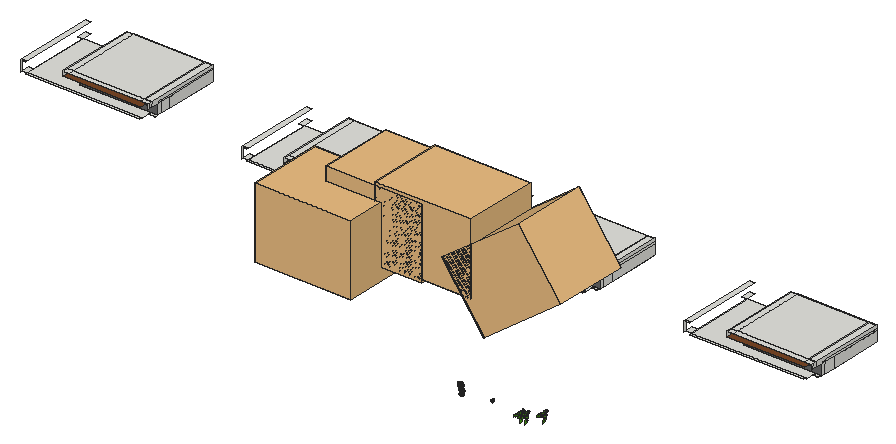
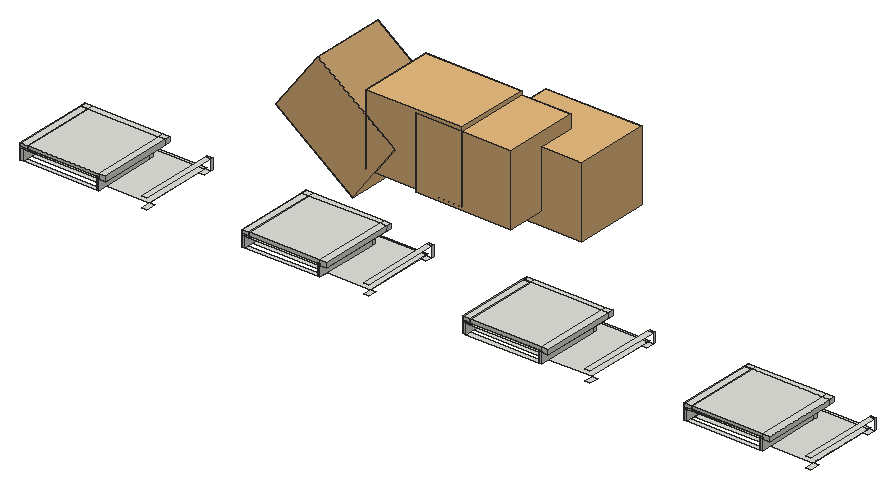
# SketchUp Ruby script. Lengths in inches.
U = 1.inch
M = Sketchup.active_model
def pt(a) = Geom::Point3d.new(a.map { |v| v * U })
def face(e, loops, mat)
  f = e.add_face(loops[0].map { |a| pt(a) })
  loops[1..].each { |l| e.add_face(l.map { |a| pt(a) }).erase! }
  f.material = f.back_material = mat if mat
  f
end
# faces: each face lists its corners as indices into pts; further lists are holes
def faces(e, pts, list, mat = nil) = list.each { |f| face(e, (f[0].is_a?(Array) ? f : [f]).map { |l| l.map { |i| pts[i] } }, mat) }
# xy, xz, yz: faces in a plane at the given z, y or x. An outline is a flat list of corners, or four numbers for a rectangle; further outlines are holes
def ring(l) = l.size == 4 ? [[l[0], l[1]], [l[2], l[1]], [l[2], l[3]], [l[0], l[3]]] : l.each_slice(2).to_a
def flat(e, list, mat, &to3) = list.each { |f| face(e, (f[0].is_a?(Array) ? f : [f]).map { |l| ring(l).map { |u, v| to3.(u, v) } }, mat) }
def xy(e, z, list, mat = nil) = flat(e, list, mat) { |x, y| [x, y, z] }
def xz(e, y, list, mat = nil) = flat(e, list, mat) { |x, z| [x, y, z] }
def yz(e, x, list, mat = nil) = flat(e, list, mat) { |y, z| [x, y, z] }
def lines(e, pts, list) = list.each { |a, b| e.add_line(pt(pts[a]), pt(pts[b])) }
# prism: a flat outline (further loops are holes) pulled along v
def prism(e, loops, v, mat = nil)
  f = face(e, loops, mat); d = Geom::Vector3d.new(v.map { |x| x * U })
  f.pushpull(f.normal.samedirection?(d) ? d.length : -d.length)
end
def box(e, o, s, mat = nil) = prism(e, [[o, [o[0] + s[0], o[1], o[2]], [o[0] + s[0], o[1] + s[1], o[2]], [o[0], o[1] + s[1], o[2]]]], [0, 0, s[2]], mat)
def at(x, y, z, deg = 0) = Geom::Transformation.translation(pt([x, y, z])) * Geom::Transformation.rotation(ORIGIN, Z_AXIS, deg.degrees)
def axes(o, x, y, z) = Geom::Transformation.new([*x, 0, *y, 0, *z, 0, *pt(o).to_a, 1])
def part(name) = M.definitions.add(name)
# library, detail: a bought-in or finely detailed component or shape, given as its bounding box
def library(name, o, s) = part(name).tap { |d| box(d.entities, o, s) }
def detail(e, o, s) = box(e.add_group.entities, o, s)
def put(e, d, t, mat = nil) = e.add_instance(d, t).tap { |i| i.material = mat if mat }
def group(e, t, mat = nil) = e.add_group.tap { |g| g.transformation = t; g.material = mat if mat }.entities
root = M.entities
M.materials.add("[Slate Light Tile]").color = [104, 104, 104]
M.materials.add("[Wood Veneer 01]").color = [120, 70, 37]
M.materials.add("hojas").color = [70, 150, 19]
c1 = part("rama-acacia")
p = [[-13.53,0.69,-1.07],[-13.38,0.86,-0.98],[-13.61,0.85,-1.06],[-14.07,0.85,-1.21],[-15.17,0.86,-1.58],[-15.95,0.92,-1.83],
  [-16.01,1,-1.83],[-16.01,1.17,-1.78],[-16.07,1.93,-1.6],[-16.4,2.73,-1.5],[-16.65,3.06,-1.5],[-17.13,4.01,-1.41],
  [-17.78,4.7,-1.44],[-18.28,5.07,-1.51],[-18.57,5.18,-1.58],[-18.91,5.47,-1.62],[-19.07,5.48,-1.67],[-19.35,5.61,-1.73],
  [-19.51,5.64,-1.78],[-19.38,5.57,-1.75],[-19.33,5.5,-1.75],[-19.31,5.23,-1.82],[-19.38,5.08,-1.89],[-19.41,4.84,-1.96],
  [-19.36,4.59,-2.01],[-19.43,4.55,-2.04],[-19.36,4.15,-2.125],[-19.21,3.7,-2.19],[-18.875,3.1,-2.24],[-18.61,2.78,-2.24],
  [-17.83,2.19,-2.13],[-17.4375,1.85,-2.09],[-17.04,1.49,-2.05],[-16.61,1.24,-1.97],[-16.17,1.0625,-1.87],[-16.06,0.95,-1.86],
  [-16.06,0.91,-1.87],[-16.32,0.9,-1.96],[-16.7,0.88,-2.1],[-17.05,0.91,-2.21],[-17.61,1.15,-2.33],[-18.06,1.29,-2.45],
  [-18.88,1.53,-2.67],[-20.25,1.46,-3.15],[-20.59,1.49,-3.26],[-20.79,1.37,-3.36],[-21.08,1.2,-3.5],[-21.28,1.22,-3.5625],
  [-21.48,0.94,-3.71],[-21.79,0.5,-3.93],[-22.02,0.17,-4.1],[-22.11,0.05,-4.16],[-22.21,-0.02,-4.21],[-22.375,-0.05,-4.28],
  [-22.375,-0.07,-4.28],[-22.18,-0.09,-4.22],[-22.11,-0.07,-4.19],[-21.78,-0.1,-4.09],[-21.6,-0.18,-4.05],[-21.52,-0.27,-4.04],
  [-21.33,-0.33,-4],[-20.94,-0.54,-3.92],[-20.6875,-0.63,-3.86],[-20.54,-0.68,-3.82],[-20.42,-0.67,-3.78],[-20.09,-0.46,-3.61],
  [-19.8,-0.24,-3.45],[-19.21,-0.02,-3.19],[-18.48,0.08,-2.92],[-17.72,0.38,-2.58],[-17.4,0.5,-2.4375],[-16.93,0.75,-2.21],
  [-16.78,0.8,-2.15],[-16.1,0.83,-1.91],[-16.0625,0.81,-1.9],[-16.08,0.77,-1.91],[-16.27,0.72,-1.99],[-16.88,0.39,-2.29],
  [-17.1875,0.15,-2.46],[-17.27,0.02,-2.52],[-17.94,-0.52,-2.89],[-17.94,-0.59,-2.91],[-18.08,-0.68,-2.99],[-18.13,-0.86,-3.05],
  [-18.56,-1.55,-3.38],[-18.71,-2.11,-3.58],[-18.79,-2.61,-3.74],[-18.86,-2.84,-3.83],[-18.87,-3.07,-3.89],[-18.84,-3.22,-3.92],
  [-18.8,-3.26,-3.92],[-18.76,-3.47,-3.96],[-18.76,-3.6,-4],[-18.67,-3.8,-4.02],[-18.61,-3.92,-4.04],[-18.58,-4.11,-4.07],
  [-18.53,-4.18,-4.08],[-18.58,-4.35,-4.14],[-18.65,-4.43,-4.18],[-18.72,-4.51,-4.23],[-18.8125,-4.51,-4.26],[-18.8125,-4.53,-4.26],
  [-18.72,-4.54,-4.24],[-18.66,-4.49,-4.21],[-18.58,-4.43,-4.16],[-18.35,-4.23,-4.03],[-18.32,-4.17,-4],[-18.22,-4.125,-3.95],
  [-18.1,-4,-3.88],[-17.79,-3.72,-3.7],[-17.68,-3.51,-3.61],[-17.32,-3.13,-3.38],[-17.24,-2.94,-3.31],[-16.78,-2.12,-2.93],
  [-16.48,-1.78,-2.73],[-16.3,-1.28,-2.54],[-16.05,-0.75,-2.3125],[-15.89,-0.2,-2.11],[-15.89,0.39,-1.95],[-15.96,0.79,-1.87],
  [-15.91,0.82,-1.84],[-15.27,0.8,-1.63],[-14.18,0.76,-1.27],[-13.78,0.73,-1.15],[-13.78,0.67,-1.16],[-14.23,0.54,-1.35],
  [-14.65,0.33,-1.55],[-14.97,0.02,-1.74],[-15.25,-0.36,-1.9375],[-15.57,-0.72,-2.14],[-15.96,-1.64,-2.52],[-16.2,-2.51,-2.84],
  [-16.2,-3.12,-3],[-16.14,-3.41,-3.06],[-16.1,-3.75,-3.14],[-16.1,-4.09,-3.23],[-16.2,-4.25,-3.3],[-16.2,-4.28,-3.3125],
  [-16.08,-4.19,-3.24],[-15.98,-4.08,-3.18],[-15.96,-3.94,-3.14],[-15.96,-3.8125,-3.1],[-15.9,-3.72,-3.06],[-15.68,-3.55,-2.9375],
  [-15.51,-3.49,-2.86],[-15.3,-3.33,-2.75],[-15.23,-3.17,-2.68],[-15.01,-3.03,-2.57],[-14.875,-2.83,-2.47],[-14.6,-2.59,-2.3125],
  [-14.4,-2.27,-2.16],[-14.12,-1.6,-1.89],[-13.91,-1.1,-1.68],[-13.67,-0.83,-1.53],[-13.53,-0.45,-1.38],[-13.53,0.67,-1.08],
  [-12.41,6.01,0.65],[-12.44,6.14,0.68],[-12.41,6.29,0.73],[-12.43,6.29,0.73],[-12.44,6.26,0.72],[-12.47,6.15,0.68],
  [-12.49,6.07,0.66],[-12.57,5.75,0.55],[-12.67,5.36,0.43],[-12.79,4.875,0.28],[-12.83,4.52,0.18],[-12.83,3.99,0.04],
  [-12.73,3.11,-0.18],[-12.58,2.52,-0.3125],[-12.3,1.97,-0.41],[-11.88,1.51,-0.46],[-11.37,1.0625,-0.48],[-10.75,0.75,-0.45],
  [-10.75,0.68,-0.47],[-12.55,0.7,-0.79],[-13.21,0.79,-0.89],[-13.2,0.67,-0.92],[-12.56,0.62,-0.82],[-11.15,0.56,-0.58],
  [-10.79,0.54,-0.52],[-10.72,0.52,-0.51],[-10.72,0.5,-0.52],[-10.87,0.47,-0.55],[-11.14,0.41,-0.62],[-11.39,0.27,-0.7],
  [-11.625,-0.01,-0.82],[-11.8,-0.43,-0.96],[-11.83,-0.57,-1],[-12.02,-1.08,-1.17],[-12.1,-1.39,-1.27],[-12.17,-1.95,-1.4375],
  [-12.17,-2.77,-1.65],[-12.09,-3.59,-1.86],[-11.86,-4.26,-2],[-11.8125,-4.4,-2.03],[-11.84,-4.49,-2.05],[-11.91,-4.6,-2.1],
  [-11.97,-4.65,-2.12],[-11.98,-4.67,-2.13],[-11.92,-4.65,-2.11],[-11.84,-4.59,-2.08],[-11.77,-4.52,-2.05],[-11.74,-4.47,-2.03],
  [-11.37,-4.3125,-1.92],[-10.95,-4.0625,-1.78],[-10.82,-3.89,-1.71],[-10.64,-3.57,-1.59],[-10.41,-3.05,-1.41],[-10.27,-2.73,-1.3],
  [-10.07,-1.88,-1.03],[-10.15,-0.71,-0.73],[-10.31,-0.1,-0.6],[-10.5,0.4,-0.5],[-10.5,0.48,-0.48],[-10.44,0.53,-0.45],
  [-10.39,0.64,-0.42],[-10.52,0.73,-0.42],[-10.44,0.93,-0.35],[-10.44,1.2,-0.28],[-10.32,1.47,-0.18],[-10.48,2.6875,0.12],
  [-10.43,2.96,0.2],[-10.75,3.87,0.38],[-11.26,4.93,0.57],[-11.8,5.54,0.64],[-12.37,5.93,0.64],[-7.78,0.19,-0.06],
  [-7.78,0.25,-0.04],[-7.75,0.39,0],[-7.89,0.4,-0.02],[-7.96,0.46,-0.02],[-7.96,0.49,-0.01],[-7.76,0.62,0.06],
  [-7.53,0.99,0.2],[-7.31,1.78,0.45],[-7.31,2.74,0.71],[-7.63,3.6875,0.9],[-8.02,4.57,1.07],[-8.66,5.23,1.13],
  [-8.83,5.4,1.14],[-8.92,5.54,1.16],[-9.1,5.64,1.16],[-9.08,5.6,1.15],[-9.02,5.56,1.15],[-8.94,5.46,1.14],
  [-8.9,5.37,1.12],[-8.9375,5.25,1.08],[-9.14,4.92,0.96],[-9.31,4.5625,0.83],[-9.39,3.73,0.6],[-9.44,2.76,0.32],
  [-9.23,1.59,0.05],[-8.82,0.9,-0.06],[-8.36,0.59,-0.0625],[-8.14,0.51,-0.04],[-8.05,0.48,-0.03],[-8.05,0.46,-0.04],
  [-8.12,0.43,-0.06],[-10.1,0.49,-0.4],[-8.22,0.3125,-0.11],[-8.22,0.25,-0.125],[-8.53,0.13,-0.21],[-8.8,-0.16,-0.34],
  [-8.96,-0.61,-0.49],[-8.96,-0.87,-0.56],[-9.16,-1.42,-0.74],[-9.13,-1.77,-0.83],[-9.09,-1.83,-0.84],[-9.125,-1.92,-0.87],
  [-9.125,-2.13,-0.93],[-9.08,-2.23,-0.95],[-9.15,-2.39,-1],[-9.11,-2.67,-1.07],[-9.03,-2.86,-1.11],[-9.07,-3.03,-1.16],
  [-8.97,-3.23,-1.19],[-8.93,-3.44,-1.24],[-8.93,-3.71,-1.32],[-8.79,-4.05,-1.38],[-8.7,-4.25,-1.42],[-8.7,-4.39,-1.46],
  [-8.76,-4.53,-1.5],[-8.77,-4.65,-1.54],[-8.64,-4.55,-1.49],[-8.27,-4.22,-1.33],[-8.1875,-4.06,-1.27],[-8.07,-3.98,-1.23],
  [-7.98,-3.79,-1.17],[-7.79,-3.59,-1.08],[-7.64,-3.3,-0.97],[-7.64,-3.25,-0.96],[-7.59,-3.21,-0.9375],[-7.52,-2.93,-0.85],
  [-7.52,-2.85,-0.83],[-7.47,-2.81,-0.81],[-7.3,-2.09,-0.59],[-7.32,-2.01,-0.57],[-7.27,-1.95,-0.54],[-7.1875,-1.57,-0.42],
  [-7.17,-1.46,-0.39],[-7.17,-1.16,-0.3125],[-7.23,-0.61,-0.17],[-7.49,-0.15,-0.1],[-13.39,-0.07,-1.23],[-13.39,0.25,-1.14],
  [-13.49,0.5625,-1.09],[-13.8,1.01,-1.08],[-13.61,0.91,-1.04],[-13.38,0.92,-0.96],[-13.32,1.03,-0.91],[-13.32,1.35,-0.82],
  [-13.28,1.49,-0.77],[-13.28,1.99,-0.64],[-13.44,2.67,-0.51],[-13.72,3.31,-0.43],[-13.93,3.71,-0.4],[-14.1,4.39,-0.27],
  [-14.5625,5.06,-0.25],[-14.89,5.62,-0.21],[-15.33,6.1,-0.23],[-15.65,6.8,-0.15],[-15.79,6.89,-0.18],[-15.61,6.52,-0.22],
  [-15.51,6.32,-0.24],[-15.45,6.28,-0.23],[-15.52,6,-0.32],[-15.63,5.6875,-0.45],[-15.77,4.97,-0.68],[-15.7,4.25,-0.85],
  [-15.46,3,-1.11],[-15,2.03,-1.21],[-14.3,1.29,-1.17],[-4.5625,0.33,0.09],[-4.22,0.49,0.13],[-4,0.7,0.1875],
  [-3.86,0.99,0.26],[-3.77,1.41,0.38],[-3.7,1.73,0.46],[-3.77,1.99,0.53],[-3.85,2.17,0.58],[-3.88,2.57,0.6875],
  [-3.98,2.9,0.78],[-4.0625,2.97,0.8],[-4.1,3.14,0.84],[-4.1875,3.25,0.87],[-4.27,3.55,0.95],[-4.31,3.71,0.99],
  [-4.42,3.9,1.04],[-4.625,4.2,1.125],[-4.72,4.39,1.18],[-4.89,4.57,1.23],[-4.98,4.73,1.27],[-5,4.72,1.26],
  [-5.01,4.51,1.21],[-4.96,4.32,1.16],[-4.97,4.27,1.14],[-5.14,3.78,1.01],[-5.3,3.39,0.91],[-5.44,2.76,0.74],
  [-5.5,2.09,0.56],[-5.57,1.78,0.48],[-5.57,1.42,0.38],[-5.57,1.09,0.29],[-5.47,0.72,0.19],[-5.22,0.44,0.12],
  [-4.93,0.27,0.07],[-4.76,0.22,0.06],[-4.76,0.18,0.05],[-4.83,0.16,0.04],[-5.26,0,0],[-5.34,-0.04,-0.01],
  [-5.47,-0.22,-0.06],[-5.51,-0.6,-0.16],[-5.42,-1.09,-0.29],[-5.28,-1.49,-0.4],[-5.21,-1.87,-0.5],[-5.11,-2.15,-0.57],
  [-5.08,-2.34,-0.63],[-5.01,-2.47,-0.66],[-4.96,-2.69,-0.72],[-4.86,-2.9375,-0.79],[-4.84,-3.07,-0.82],[-4.77,-3.18,-0.85],
  [-4.74,-3.43,-0.92],[-4.7,-3.71,-0.99],[-4.62,-3.89,-1.04],[-4.58,-3.98,-1.07],[-4.58,-3.83,-1.03],[-4.51,-3.67,-0.98],
  [-4.3,-3.32,-0.89],[-4.16,-3.09,-0.83],[-4.16,-2.98,-0.8],[-4.11,-2.92,-0.78],[-4.02,-2.8,-0.75],[-3.95,-2.59,-0.69],
  [-3.95,-2.33,-0.625],[-3.86,-2.26,-0.6],[-3.86,-2.02,-0.54],[-3.86,-1.44,-0.39],[-3.94,-1.22,-0.33],[-3.94,-1.08,-0.29],
  [-4,-0.96,-0.26],[-4,-0.87,-0.23],[-4.0625,-0.8125,-0.22],[-4.16,-0.54,-0.14],[-4.39,-0.24,-0.06],[-4.61,-0.08,-0.02],
  [-4.77,-0.03,-0.01],[-4.77,-0.01,0],[-4.65,-0.01,0],[-4.61,0.19,0.05],[-4.66,0.23,0.0625],[-4.63,0.29,0.08],
  [-4.07,0.17,0.04],[0,-0.24,-0.06],[0,0,0],[-0.5,0.04,0.01],[-1.58,0.08,0.02],[-13.78,0.67,-1.08]]
faces(c1.entities,p,[[0,1,2,3,4,5,6,7,8,9,10,11,12,13,14,15,16,17,18,19,20,21,22,23,24,25,26,27,28,29,30,31,32,33,34,35,36,37,38,39,40,41,42,43,44,45,46,47,48,49,50,51,52,53,54,55,56,57,58,59,60,61,62,63,64,65,66,67,68,69,70,71,72,73,74,75,76,77,78,79,80,81,82,83,84,85,86,87,88,89,90,91,92,93,94,95,96,97,98,99,100,101,102,103,104,105,106,107,108,109,110,111,112,113,114,115,116,117,118,119,120,121,122,123,124,125,126,127,128,129,130,131,132,133,134,135,136,137,138,139,140,141,142,143,144,145,146,147,148,149,150,151,152,153,154,155],[156,157,158,159,160,161,162,163,164,165,166,167,168,169,170,171,172,173,174,175,176,177,178,179,180,181,182,183,184,185,186,187,188,189,190,191,192,193,194,195,196,197,198,199,200,201,202,203,204,205,206,207,208,209,210,211,212,213,214,215,216,217,218,219,220,221,222,223,224,225,226],[227,228,229,230,231,232,233,234,235,236,237,238,239,240,241,242,243,244,245,246,247,248,249,250,251,252,253,254,255,256,257,258,216,215,259,260,261,262,263,264,265,266,267,268,269,270,271,272,273,274,275,276,277,278,279,280,281,282,283,284,285,286,287,288,289,290,291,292,293,294,295,296,297,298,299,300,301,302,303],[154,304,305,306,155],[307,308,1,309,310,311,312,313,314,315,316,317,318,319,320,321,322,323,324,325,326,327,328,329,330,331,332],[333,334,335,336,337,338,339,340,341,342,343,344,345,346,347,348,349,350,351,352,353,354,355,356,357,358,359,360,361,362,363,364,365,366,367,368,369,370,371,372,373,374,375,376,377,378,379,380,381,382,383,384,385,386,387,388,389,390,391,392,393,394,395,396,397,398,399,400,401,402,403,404,405,406,407,408,409,410,411,412,413],[0,177,1],[308,2,1],
  [176,1,177],[414,411,410,415,416,417,418],[228,370,229],[369,229,370]],"hojas")
lines(c1.entities,p,[[155,419]])
c2 = part("Group\#150")
put(c2.entities,c1,axes([10.13,10.27,0],[0.45315,0.21131,0],[-0.21131,0.45315,0],[0,0,0.5]))
put(c2.entities,c1,axes([10.13,10.27,0],[0.11638,0.47539,0.10227],[-0.48087,0.12813,-0.0484],[-0.07223,-0.08709,0.48703]))
put(c2.entities,c1,axes([9.58,10.26,-0.7],[0.1449,0.38901,-0.2787],[-0.10883,0.31035,0.37662],[0.46601,-0.04848,0.17461]))
c3 = part("Group\#151")
put(c3.entities,c2,axes([24.99,4.24,9.59],[0.78856,0.61496,0],[0.01473,-0.01889,0.99971],[0.61478,-0.78833,-0.02396]))
put(c3.entities,c2,axes([39.5,6.625,12.55],[0.6544,0.49291,0.57341],[-0.44023,-0.3682,0.81892],[0.61478,-0.78833,-0.02396]))
put(c3.entities,c2,axes([32.34,3.7,6.88],[0.78856,0.61496,0],[0.01473,-0.01889,0.99971],[0.61478,-0.78833,-0.02396]))
put(c3.entities,c2,axes([43.14,6.65,17.54],[0.78856,0.61496,0],[0.35273,-0.4523,0.81915],[0.50374,-0.64595,-0.57358]))
put(c3.entities,c2,axes([12.2,6.2,16.68],[0.7209,0.54936,0.4225],[-0.31991,-0.27701,0.90605],[0.61478,-0.78833,-0.02396]))
put(c3.entities,c2,axes([49.9375,3.79,26.09],[0.78856,0.61496,0],[0.01473,-0.01889,0.99971],[0.61478,-0.78833,-0.02396]))
put(c3.entities,c2,axes([36.11,4.9375,33.94],[0.78856,0.61496,0],[0.01473,-0.01889,0.99971],[0.61478,-0.78833,-0.02396]))
put(c3.entities,c2,axes([39.61,3.79,23.47],[0.78856,0.61496,0],[0.01473,-0.01889,0.99971],[0.61478,-0.78833,-0.02396]))
put(c3.entities,c2,axes([25.59,6.5625,46.47],[-0.40704,-0.29112,-0.86578],[0.67555,0.54201,-0.49986],[0.61478,-0.78833,-0.02396]))
put(c3.entities,c2,axes([54.97,1.98,11.65],[0.78856,0.61496,0],[0.01473,-0.01889,0.99971],[0.61478,-0.78833,-0.02396]))
put(c3.entities,c2,axes([32.97,3.79,19.14],[0.78856,0.61496,0],[0.01473,-0.01889,0.99971],[0.61478,-0.78833,-0.02396]))
put(c3.entities,c2,axes([24.24,3.79,21.99],[0.78856,0.61496,0],[0.01473,-0.01889,0.99971],[0.61478,-0.78833,-0.02396]))
put(c3.entities,c2,axes([16.86,4.24,12.3],[0.78856,0.61496,0],[0.01473,-0.01889,0.99971],[0.61478,-0.78833,-0.02396]))
put(c3.entities,c2,axes([1.23,3.9375,19.07],[0.78856,0.61496,0],[0.01473,-0.01889,0.99971],[0.61478,-0.78833,-0.02396]))
put(c3.entities,c2,axes([29.05,5.25,29.11],[0.78856,0.61496,0],[0.21033,-0.2697,0.93969],[0.57787,-0.741,-0.34202]))
put(c3.entities,c2,axes([24.16,3.79,-0.1],[0.78856,0.61496,0],[0.01473,-0.01889,0.99971],[0.61478,-0.78833,-0.02396]))
c4 = library("Sans+titre+(1)+(1)+(2)",[-30.91,-35.46,0],[63.51,67.02,85.79])
xy(root,282.75,[[374.86,837.03,827.91,845.35],[1254.81,837.03,1707.86,845.35],[2134.75,837.03,2587.8,845.35],[3014.7,837.03,3467.75,845.35],[352.17,845.35,372.92,877.14],
  [374.86,845.35,827.91,845.35,827.91,846.1,832,846.1,832,877.51,857.125,877.51,857.125,890.39,545.16,890.39,545.16,1122.97,374.86,1122.97],[827.91,845.35,832,846.1],[1232.12,845.35,1252.87,877.14],[1254.81,845.35,1707.86,845.35,1707.86,846.1,1711.94,846.1,1711.94,877.51,1737.07,877.51,1737.07,890.39,1425.1,890.39,1425.1,1122.97,1254.81,1122.97],[1707.86,845.35,1711.94,846.1],
  [2112.0625,845.35,2132.8125,877.14],[2134.75,845.35,2587.8,845.35,2587.8,846.1,2591.89,846.1,2591.89,877.51,2617.01,877.51,2617.01,890.39,2305.05,890.39,2305.05,1122.97,2134.75,1122.97],[2587.8,845.35,2591.89,846.1],[2992.01,845.35,3012.76,877.14],[3014.7,845.35,3467.75,845.35,3467.75,846.1,3471.83,846.1,3471.83,877.51,3496.96,877.51,3496.96,890.39,3184.99,890.39,3184.99,1122.97,3014.7,1122.97],
  [3467.75,845.35,3471.83,846.1],[372.92,850.97,374.86,1122.97],[1252.87,850.97,1254.81,1122.97],[2132.8125,850.97,2134.75,1122.97],[3012.76,850.97,3014.7,1122.97],
  [832,877.14,857.125,877.51],[1711.94,877.14,1737.07,877.51],[2591.89,877.14,2617.01,877.51],[3471.83,877.14,3496.96,877.51],[545.16,890.39,857.125,905.7],
  [1425.1,890.39,1737.07,905.7],[2305.05,890.39,2617.01,905.7],[3184.99,890.39,3496.96,905.7],[545.16,905.7,554.54,1122.97],[554.54,905.7,844.86,1122.97],
  [844.86,905.7,857.125,947.51],[1425.1,905.7,1434.48,1122.97],[1434.48,905.7,1724.81,1122.97],[1724.81,905.7,1737.07,947.51],[2305.05,905.7,2314.43,1122.97],
  [2314.43,905.7,2604.75,1122.97],[2604.75,905.7,2617.01,947.51],[3184.99,905.7,3194.375,1122.97],[3194.375,905.7,3484.69,1122.97],[3484.69,905.7,3496.96,947.51],
  [844.86,947.51,857.125,1122.97],[1724.81,947.51,1737.07,1122.97],[2604.75,947.51,2617.01,1122.97],[3484.69,947.51,3496.96,1122.97],[352.17,1122.97,372.3,1160.85],
  [545.16,1122.97,554.54,1160.85],[844.86,1122.97,857.125,1160.85],[1232.12,1122.97,1252.24,1160.85],[1425.1,1122.97,1434.48,1160.85],[1724.81,1122.97,1737.07,1160.85],
  [2112.0625,1122.97,2132.1875,1160.85],[2305.05,1122.97,2314.43,1160.85],[2604.75,1122.97,2617.01,1160.85],[2992.01,1122.97,3012.13,1160.85],[3184.99,1122.97,3194.375,1160.85],
  [3484.69,1122.97,3496.96,1160.85],[554.54,1143.26,844.86,1160.85],[1434.48,1143.26,1724.81,1160.85],[2314.43,1143.26,2604.75,1160.85],[3194.375,1143.26,3484.69,1160.85]])
xy(root,324.5625,[[352.17,837.03,372.92,845.35],[1232.12,837.03,1252.87,845.35],[2112.0625,837.03,2132.8125,845.35],[2992.01,837.03,3012.76,845.35],[352.17,845.35,372.92,1160.85],
  [1232.12,845.35,1252.87,1160.85],[2112.0625,845.35,2132.8125,1160.85],[2992.01,845.35,3012.76,1160.85],[827.91,861.24,857.125,890.39],[1707.86,861.24,1737.07,890.39],
  [2587.8,861.24,2617.01,890.39],[3467.75,861.24,3496.96,890.39],[545.16,890.39,827.91,905.7],[827.91,890.39,857.125,905.7],[1425.1,890.39,1707.86,905.7],
  [1707.86,890.39,1737.07,905.7],[2305.05,890.39,2587.8,905.7],[2587.8,890.39,2617.01,905.7],[3184.99,890.39,3467.75,905.7],[3467.75,890.39,3496.96,905.7],
  [545.16,905.7,554.54,1160.85],[554.54,905.7,827.91,1160.85],[827.91,905.7,844.86,1160.85],[1425.1,905.7,1434.48,1160.85],[1434.48,905.7,1707.86,1160.85],
  [1707.86,905.7,1724.81,1160.85],[2305.05,905.7,2314.43,1160.85],[2314.43,905.7,2587.8,1160.85],[2587.8,905.7,2604.75,1160.85],[3184.99,905.7,3194.375,1160.85],
  [3194.375,905.7,3467.75,1160.85],[3467.75,905.7,3484.69,1160.85],[844.86,947.51,857.125,1160.85],[1724.81,947.51,1737.07,1160.85],[2604.75,947.51,2617.01,1160.85],
  [3484.69,947.51,3496.96,1160.85]])
xy(root,324.5625,[[518.47,840.97,518.47,1160.85,545.16,1160.85,545.16,890.39,827.91,890.39,827.91,840.97],[1398.41,840.97,1398.41,1160.85,1425.1,1160.85,1425.1,890.39,1707.86,890.39,1707.86,840.97],[2278.36,840.97,2278.36,1160.85,2305.05,1160.85,2305.05,890.39,2587.8,890.39,2587.8,840.97],[3158.3,840.97,3158.3,1160.85,3184.99,1160.85,3184.99,890.39,3467.75,890.39,3467.75,840.97]],"[Wood Veneer 01]")
xy(root,331.1875,[[545.16,890.39,857.125,905.7],[1425.1,890.39,1737.07,905.7],[2305.05,890.39,2617.01,905.7],[3184.99,890.39,3496.96,905.7],[545.16,905.7,554.54,1160.85],
  [554.54,905.7,844.86,1160.85],[844.86,905.7,857.125,1160.85],[1425.1,905.7,1434.48,1160.85],[1434.48,905.7,1724.81,1160.85],[1724.81,905.7,1737.07,1160.85],
  [2305.05,905.7,2314.43,1160.85],[2314.43,905.7,2604.75,1160.85],[2604.75,905.7,2617.01,1160.85],[3184.99,905.7,3194.375,1160.85],[3194.375,905.7,3484.69,1160.85],
  [3484.69,905.7,3496.96,1160.85]])
xy(root,343.4375,[[518.47,840.97,545.16,861.24],[545.16,840.97,827.91,861.24],[827.91,840.97,857.125,861.24],[1398.41,840.97,1425.1,861.24],[1425.1,840.97,1707.86,861.24],
  [1707.86,840.97,1737.07,861.24],[2278.36,840.97,2305.05,861.24],[2305.05,840.97,2587.8,861.24],[2587.8,840.97,2617.01,861.24],[3158.3,840.97,3184.99,861.24],
  [3184.99,840.97,3467.75,861.24],[3467.75,840.97,3496.96,861.24],[518.47,861.24,545.16,1160.85],[545.16,861.24,827.91,1160.85],[827.91,861.24,857.125,1160.85],
  [1398.41,861.24,1425.1,1160.85],[1425.1,861.24,1707.86,1160.85],[1707.86,861.24,1737.07,1160.85],[2278.36,861.24,2305.05,1160.85],[2305.05,861.24,2587.8,1160.85],
  [2587.8,861.24,2617.01,1160.85],[3158.3,861.24,3184.99,1160.85],[3184.99,861.24,3467.75,1160.85],[3467.75,861.24,3496.96,1160.85]])
xz(root,861.24,[[827.91,324.5625,857.125,343.4375],[1707.86,324.5625,1737.07,343.4375],[2587.8,324.5625,2617.01,343.4375],[3467.75,324.5625,3496.96,343.4375]])
xz(root,890.39,[[545.16,324.5625,857.125,331.1875],[1425.1,324.5625,1737.07,331.1875],[2305.05,324.5625,2617.01,331.1875],[3184.99,324.5625,3496.96,331.1875]])
xz(root,890.39,[[545.16,282.75,857.125,324.5625],[1425.1,282.75,1737.07,324.5625],[2305.05,282.75,2617.01,324.5625],[3184.99,282.75,3496.96,324.5625]],"[Slate Light Tile]")
xz(root,905.7,[[545.16,282.75,554.54,324.5625],[554.54,282.75,844.86,324.5625],[844.86,282.75,857.125,324.5625],[1425.1,282.75,1434.48,324.5625],[1434.48,282.75,1724.81,324.5625],
  [1724.81,282.75,1737.07,324.5625],[2305.05,282.75,2314.43,324.5625],[2314.43,282.75,2604.75,324.5625],[2604.75,282.75,2617.01,324.5625],[3184.99,282.75,3194.375,324.5625],
  [3194.375,282.75,3484.69,324.5625],[3484.69,282.75,3496.96,324.5625],[545.16,324.5625,554.54,331.1875],[554.54,324.5625,844.86,331.1875],[844.86,324.5625,857.125,331.1875],
  [1425.1,324.5625,1434.48,331.1875],[1434.48,324.5625,1724.81,331.1875],[1724.81,324.5625,1737.07,331.1875],[2305.05,324.5625,2314.43,331.1875],[2314.43,324.5625,2604.75,331.1875],
  [2604.75,324.5625,2617.01,331.1875],[3184.99,324.5625,3194.375,331.1875],[3194.375,324.5625,3484.69,331.1875],[3484.69,324.5625,3496.96,331.1875]])
xz(root,947.51,[[844.86,282.75,857.125,324.5625],[1724.81,282.75,1737.07,324.5625],[2604.75,282.75,2617.01,324.5625],[3484.69,282.75,3496.96,324.5625]])
xz(root,1160.85,[[545.16,282.75,554.54,324.5625],[844.86,282.75,857.125,324.5625],[1425.1,282.75,1434.48,324.5625],[1724.81,282.75,1737.07,324.5625],[2305.05,282.75,2314.43,324.5625],
  [2604.75,282.75,2617.01,324.5625],[3184.99,282.75,3194.375,324.5625],[3484.69,282.75,3496.96,324.5625],[518.47,324.5625,545.16,343.4375],[545.16,324.5625,554.54,331.1875],
  [827.91,324.5625,844.86,331.1875],[844.86,324.5625,857.125,331.1875],[1398.41,324.5625,1425.1,343.4375],[1425.1,324.5625,1434.48,331.1875],[1707.86,324.5625,1724.81,331.1875],
  [1724.81,324.5625,1737.07,331.1875],[2278.36,324.5625,2305.05,343.4375],[2305.05,324.5625,2314.43,331.1875],[2587.8,324.5625,2604.75,331.1875],[2604.75,324.5625,2617.01,331.1875],
  [3158.3,324.5625,3184.99,343.4375],[3184.99,324.5625,3194.375,331.1875],[3467.75,324.5625,3484.69,331.1875],[3484.69,324.5625,3496.96,331.1875],[545.16,331.1875,827.91,343.4375],
  [827.91,331.1875,857.125,343.4375],[1425.1,331.1875,1707.86,343.4375],[1707.86,331.1875,1737.07,343.4375],[2305.05,331.1875,2587.8,343.4375],[2587.8,331.1875,2617.01,343.4375],
  [3184.99,331.1875,3467.75,343.4375],[3467.75,331.1875,3496.96,343.4375]])
yz(root,352.17,[[837.03,282.75,845.35,324.5625]])
yz(root,518.47,[[840.97,324.5625,861.24,343.4375],[861.24,324.5625,1160.85,343.4375]])
yz(root,545.16,[[890.39,282.75,905.7,324.5625],[905.7,282.75,1160.85,324.5625],[890.39,324.5625,905.7,331.1875],[905.7,324.5625,1160.85,331.1875]])
yz(root,554.54,[[905.7,282.75,1160.85,324.5625],[905.7,324.5625,1160.85,331.1875]])
yz(root,827.91,[[861.24,324.5625,1160.85,343.4375]])
yz(root,844.86,[[905.7,282.75,947.51,324.5625],[947.51,282.75,1160.85,324.5625],[905.7,324.5625,1160.85,331.1875]])
yz(root,857.125,[[890.39,282.75,905.7,324.5625],[905.7,282.75,947.51,324.5625],[947.51,282.75,1160.85,324.5625],[840.97,324.5625,846.1,343.4375],[846.1,324.5625,861.24,343.4375],
  [861.24,324.5625,890.39,324.5625,890.39,331.1875,1160.85,331.1875,1160.85,343.4375,861.24,343.4375],[890.39,324.5625,905.7,331.1875],[905.7,324.5625,1160.85,331.1875]])
yz(root,1232.12,[[837.03,282.75,845.35,324.5625]])
yz(root,1398.41,[[840.97,324.5625,861.24,343.4375],[861.24,324.5625,1160.85,343.4375]])
yz(root,1425.1,[[890.39,282.75,905.7,324.5625],[905.7,282.75,1160.85,324.5625],[890.39,324.5625,905.7,331.1875],[905.7,324.5625,1160.85,331.1875]])
yz(root,1434.48,[[905.7,282.75,1160.85,324.5625],[905.7,324.5625,1160.85,331.1875]])
yz(root,1707.86,[[861.24,324.5625,1160.85,343.4375]])
yz(root,1724.81,[[905.7,282.75,947.51,324.5625],[947.51,282.75,1160.85,324.5625],[905.7,324.5625,1160.85,331.1875]])
yz(root,1737.07,[[890.39,282.75,905.7,324.5625],[905.7,282.75,947.51,324.5625],[947.51,282.75,1160.85,324.5625],[840.97,324.5625,846.1,343.4375],[846.1,324.5625,861.24,343.4375],
  [861.24,324.5625,890.39,324.5625,890.39,331.1875,1160.85,331.1875,1160.85,343.4375,861.24,343.4375],[890.39,324.5625,905.7,331.1875],[905.7,324.5625,1160.85,331.1875]])
yz(root,2112.0625,[[837.03,282.75,845.35,324.5625]])
yz(root,2278.36,[[840.97,324.5625,861.24,343.4375],[861.24,324.5625,1160.85,343.4375]])
yz(root,2305.05,[[890.39,282.75,905.7,324.5625],[905.7,282.75,1160.85,324.5625],[890.39,324.5625,905.7,331.1875],[905.7,324.5625,1160.85,331.1875]])
yz(root,2314.43,[[905.7,282.75,1160.85,324.5625],[905.7,324.5625,1160.85,331.1875]])
yz(root,2587.8,[[861.24,324.5625,1160.85,343.4375]])
yz(root,2604.75,[[905.7,282.75,947.51,324.5625],[947.51,282.75,1160.85,324.5625],[905.7,324.5625,1160.85,331.1875]])
yz(root,2617.01,[[890.39,282.75,905.7,324.5625],[905.7,282.75,947.51,324.5625],[947.51,282.75,1160.85,324.5625],[840.97,324.5625,846.1,343.4375],[846.1,324.5625,861.24,343.4375],
  [861.24,324.5625,890.39,324.5625,890.39,331.1875,1160.85,331.1875,1160.85,343.4375,861.24,343.4375],[890.39,324.5625,905.7,331.1875],[905.7,324.5625,1160.85,331.1875]])
yz(root,2992.01,[[837.03,282.75,845.35,324.5625]])
yz(root,3158.3,[[840.97,324.5625,861.24,343.4375],[861.24,324.5625,1160.85,343.4375]])
yz(root,3184.99,[[890.39,282.75,905.7,324.5625],[905.7,282.75,1160.85,324.5625],[890.39,324.5625,905.7,331.1875],[905.7,324.5625,1160.85,331.1875]])
yz(root,3194.375,[[905.7,282.75,1160.85,324.5625],[905.7,324.5625,1160.85,331.1875]])
yz(root,3467.75,[[861.24,324.5625,1160.85,343.4375]])
yz(root,3484.69,[[905.7,282.75,947.51,324.5625],[947.51,282.75,1160.85,324.5625],[905.7,324.5625,1160.85,331.1875]])
yz(root,3496.96,[[890.39,282.75,905.7,324.5625],[905.7,282.75,947.51,324.5625],[947.51,282.75,1160.85,324.5625],[840.97,324.5625,846.1,343.4375],[846.1,324.5625,861.24,343.4375],
  [861.24,324.5625,890.39,324.5625,890.39,331.1875,1160.85,331.1875,1160.85,343.4375,861.24,343.4375],[890.39,324.5625,905.7,331.1875],[905.7,324.5625,1160.85,331.1875]])
p = [[2305.05,861.24,324.5625],[2305.05,861.24,343.4375],[3184.99,861.24,324.5625],[3184.99,861.24,343.4375],[545.16,861.24,324.5625],[545.16,861.24,343.4375],
  [1425.1,861.24,324.5625],[1425.1,861.24,343.4375]]
lines(root,p,[[0,1],[2,3],[4,5],[6,7]])
put(root,c2,axes([2960.57,55.24,286.61],[0.37045,4.09667,0],[0.08998,-0.06733,3.00354],[3.7549,-2.80958,-0.07198]))
put(root,c3,at(2672.47,105.37,285.28,-40))
put(root,c4,axes([2759.94,572.03,625.81],[-2.63478,0,3.57373],[0,4.44,0],[-3.57373,0,-2.63478]))
put(root,c2,axes([3010.56,83.74,295.36],[0.37045,4.09667,0],[0.08998,-0.06733,3.00354],[3.7549,-2.80958,-0.07198]))
put(root,c2,axes([2960.71,32.01,302.65],[0.37045,4.09667,0],[0.08998,-0.06733,3.00354],[3.7549,-2.80958,-0.07198]))
put(root,c2,axes([2822.08,88.97,300.12],[0.20879,0.97796,0],[0.02343,-0.005,0.99971],[0.97768,-0.20873,-0.02396]))
put(root,c4,axes([1742.31,423.74,489.3],[0,0,-4.44],[0,4.44,0],[4.44,0,0]))
put(root,c4,axes([1904.26,572.03,540.29],[0,0,-4.44],[0,4.44,0],[4.44,0,0]))
put(root,c4,axes([2101.51,572.03,554.28],[0,0,-4.44],[0,4.44,0],[4.44,0,0]))
